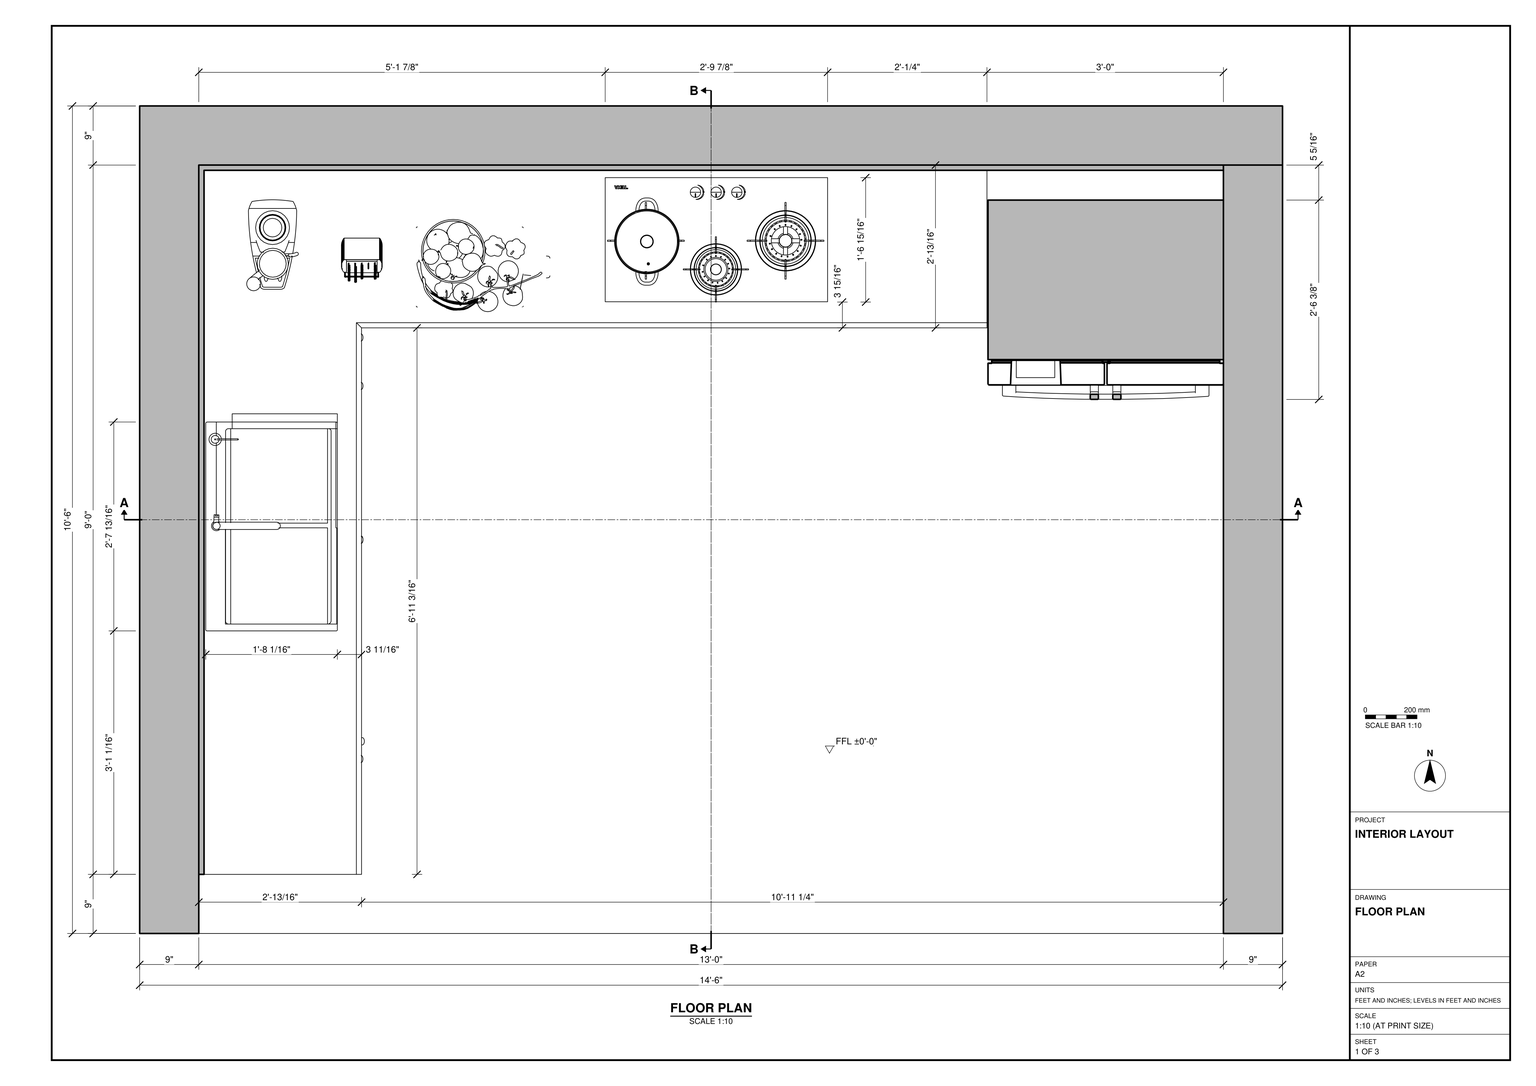
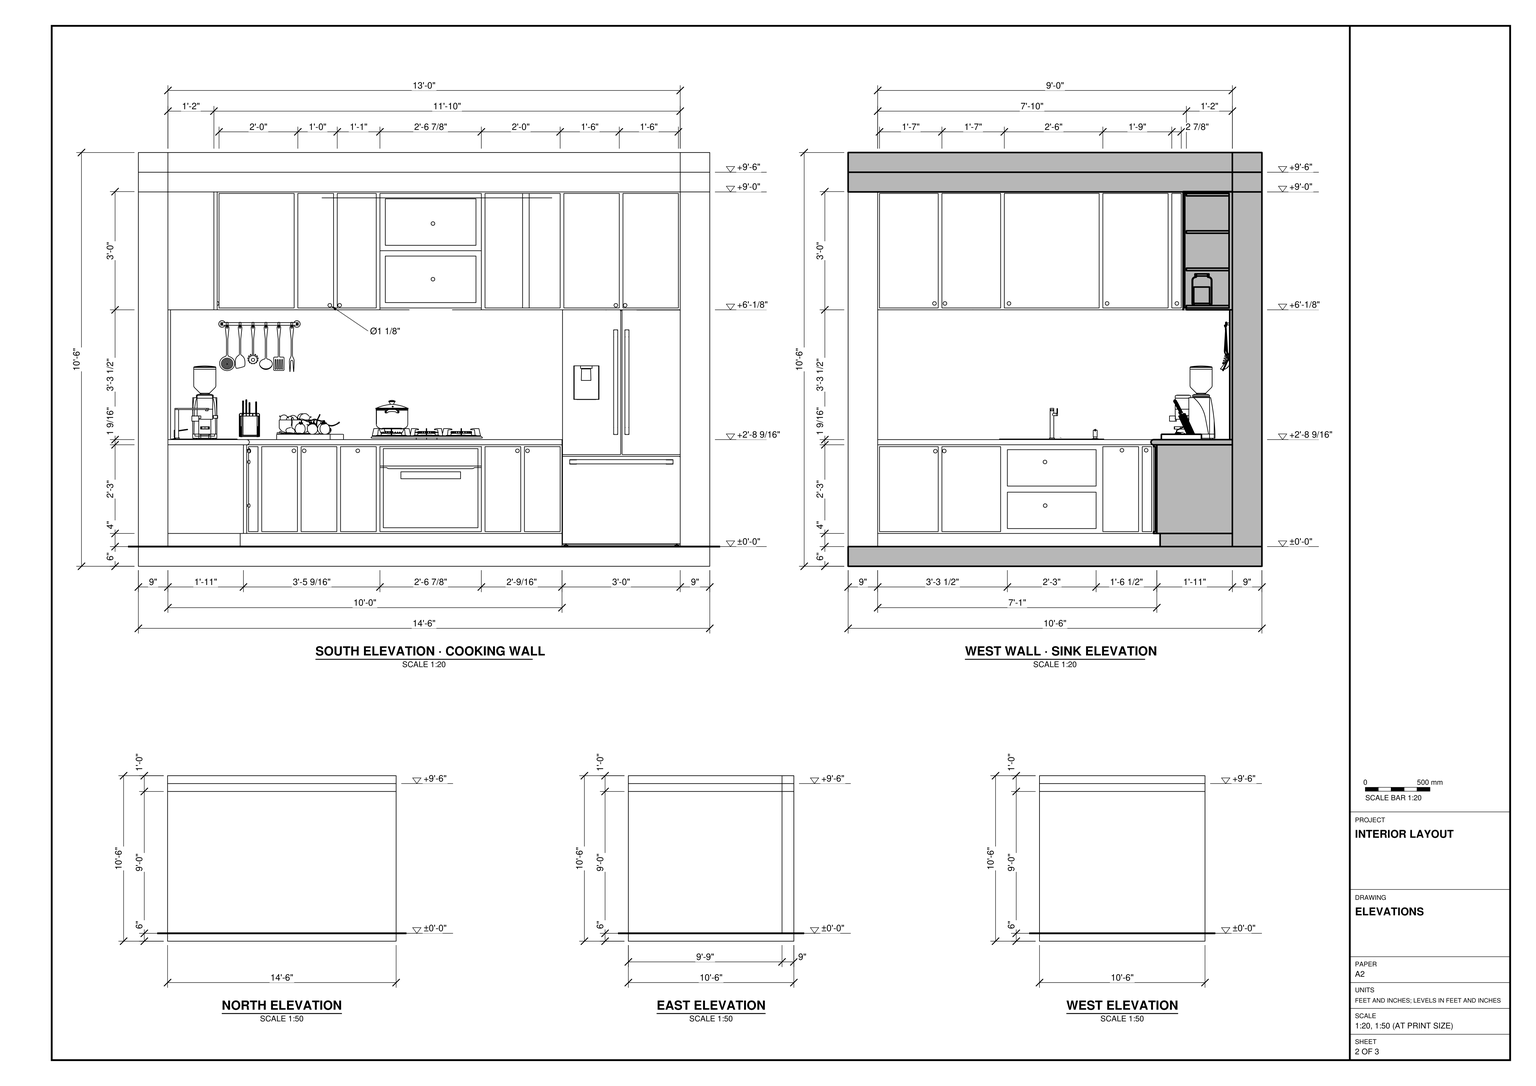
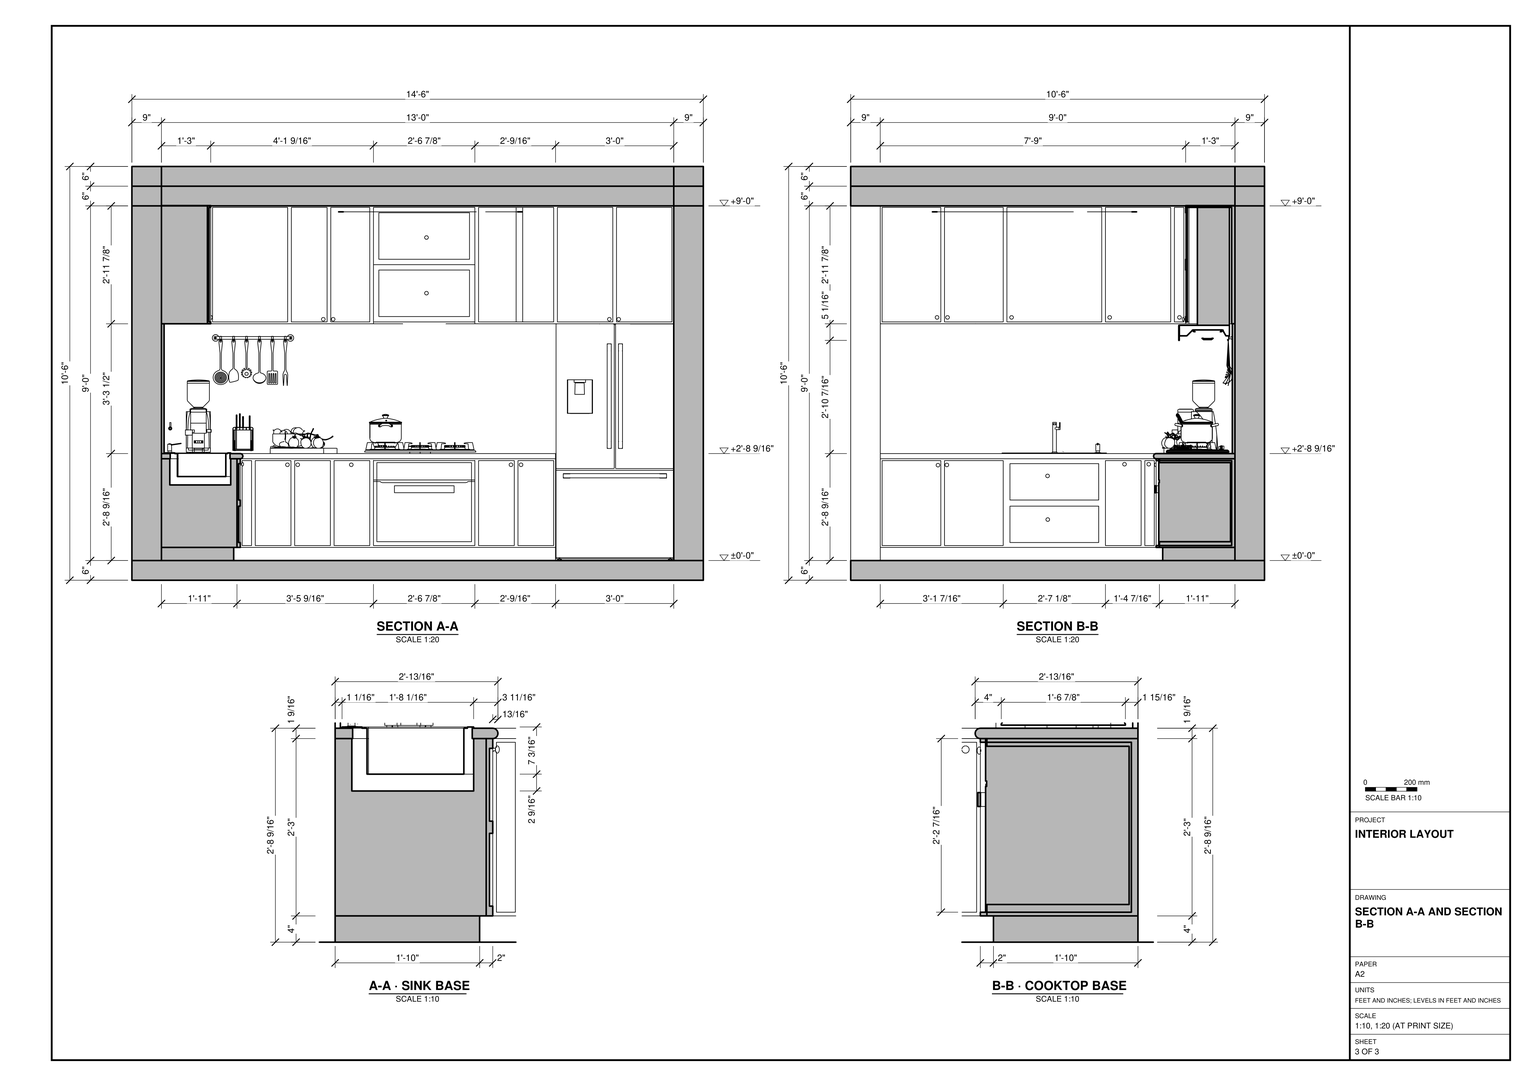
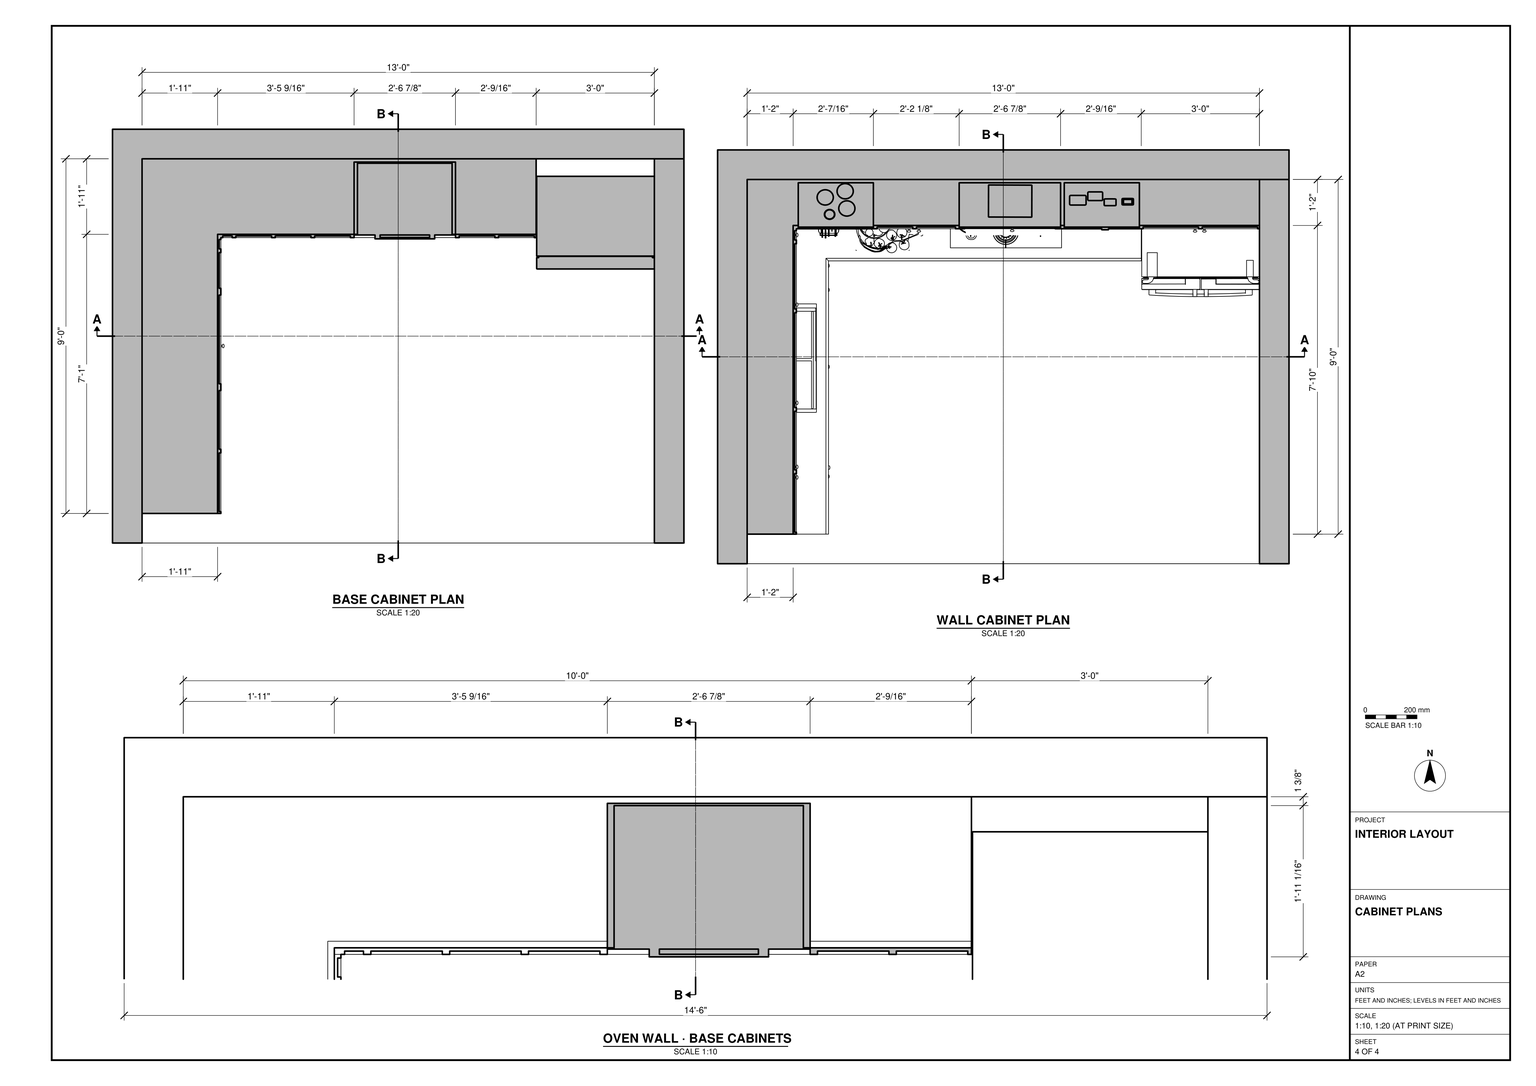
Build the kitchen interior in SketchUp from task_files/diagram_01.pdf. Work in feet and inches. The overall model is 14'-6" wide, 10'-6" deep and 10'-6" high, with the finished floor at ±0'-0". Model the floor slab, the 9" walls and the overhead slab as shown in section. Leave the front open as shown in plan.

Fit an L-shaped worktop along the cooking wall and the left-hand sink wall, leaving the middle of the room clear. Set the double-bowl sink and faucet into the return. On the cooking wall, place the cooktop over the built-in oven and end the run with the refrigerator on the right. Follow the elevations for the widths and arrangement of cabinet doors, drawer fronts and overhead cupboards, including the cupboard above the refrigerator. Use the enlarged sections for the worktop edges, cabinet depths and recessed plinths.

Decor and loose items, including appliances, cookware and counter accessories, may be any suitable library components placed as shown. Keep the shell elements and each furniture or joinery piece in separate groups or components, and use components for repeated parts. Save one SketchUp model as output_files/l_shaped_kitchen_with_fitted_cabinetry_and_appliances.skp.

# SketchUp Ruby script. Lengths in inches.
U = 1.inch
M = Sketchup.active_model
def pt(a) = Geom::Point3d.new(a.map { |v| v * U })
def face(e, loops, mat)
  f = e.add_face(loops[0].map { |a| pt(a) })
  loops[1..].each { |l| e.add_face(l.map { |a| pt(a) }).erase! }
  f.material = f.back_material = mat if mat
  f
end
# faces: each face lists its corners as indices into pts; further lists are holes
def faces(e, pts, list, mat = nil) = list.each { |f| face(e, (f[0].is_a?(Array) ? f : [f]).map { |l| l.map { |i| pts[i] } }, mat) }
# xy, xz, yz: faces in a plane at the given z, y or x. An outline is a flat list of corners, or four numbers for a rectangle; further outlines are holes
def ring(l) = l.size == 4 ? [[l[0], l[1]], [l[2], l[1]], [l[2], l[3]], [l[0], l[3]]] : l.each_slice(2).to_a
def flat(e, list, mat, &to3) = list.each { |f| face(e, (f[0].is_a?(Array) ? f : [f]).map { |l| ring(l).map { |u, v| to3.(u, v) } }, mat) }
def xy(e, z, list, mat = nil) = flat(e, list, mat) { |x, y| [x, y, z] }
def xz(e, y, list, mat = nil) = flat(e, list, mat) { |x, z| [x, y, z] }
def yz(e, x, list, mat = nil) = flat(e, list, mat) { |y, z| [x, y, z] }
def lines(e, pts, list) = list.each { |a, b| e.add_line(pt(pts[a]), pt(pts[b])) }
# prism: a flat outline (further loops are holes) pulled along v
def prism(e, loops, v, mat = nil)
  f = face(e, loops, mat); d = Geom::Vector3d.new(v.map { |x| x * U })
  f.pushpull(f.normal.samedirection?(d) ? d.length : -d.length)
end
def box(e, o, s, mat = nil) = prism(e, [[o, [o[0] + s[0], o[1], o[2]], [o[0] + s[0], o[1] + s[1], o[2]], [o[0], o[1] + s[1], o[2]]]], [0, 0, s[2]], mat)
def at(x, y, z, deg = 0) = Geom::Transformation.translation(pt([x, y, z])) * Geom::Transformation.rotation(ORIGIN, Z_AXIS, deg.degrees)
def axes(o, x, y, z) = Geom::Transformation.new([*x, 0, *y, 0, *z, 0, *pt(o).to_a, 1])
def part(name) = M.definitions.add(name)
# library, detail: a bought-in or finely detailed component or shape, given as its bounding box
def library(name, o, s) = part(name).tap { |d| box(d.entities, o, s) }
def detail(e, o, s) = box(e.add_group.entities, o, s)
def put(e, d, t, mat = nil) = e.add_instance(d, t).tap { |i| i.material = mat if mat }
def group(e, t, mat = nil) = e.add_group.tap { |g| g.transformation = t; g.material = mat if mat }.entities
root = M.entities
M.materials.add("2037 AP 8775 ROCK CRYSTAL").color = [151, 134, 122]
M.materials.add("Crazing Tile_ Stack (YETCY4)").color = [230, 230, 227]
M.materials.add("Granite (R3V8QC)").color = [36, 36, 36]
M.materials.add("Grey Victorian Tile Stack 912 x 912 mm (XTX9T6)").color = [186, 184, 188]
M.materials.add("H 6800 BM").color = [58, 58, 58]
M.materials.add("LED_3200k\#1").color = [255, 192, 121]
M.materials.add("OJ0111").color = [63, 63, 63]
M.materials.add("OJ0113").color = [243, 243, 243]
M.materials.add("OJ0114").color = [42, 42, 42]
M.materials.add("Porphyritic Granite (I3ZB3U)").color = [204, 204, 204]
M.materials.add("[Color A02]").color = [134, 143, 158]
M.materials.add("[Color M01]").color = [226, 226, 226]
M.materials.add("[Translucent Glass Gray]").color = [128, 128, 128]
M.materials["[Translucent Glass Gray]"].alpha = 0.5
c1 = library("H 6800 BM",[0,-1.38,0],[23.62,23.03,17.72])
c2 = part("Component")
xy(c2.entities,-0.07,[[484.96,-0.56,484.96,6.6,485.72,-0.48],[485.72,-0.48,484.96,6.6,486.42,-0.24],[486.42,-0.24,484.96,6.6,487.04,0.14],[487.04,0.14,484.96,6.6,487.55,0.63],[487.55,0.63,484.96,6.6,487.95,1.22],
  [487.95,1.22,484.96,6.6,488.2,1.88],[488.2,1.88,484.96,6.6,488.29,2.61],[488.29,2.61,484.96,6.6,488.29,3.43],[488.29,3.43,484.96,6.6,485.72,6.51],[488.29,3.43,485.72,6.51,488.2,4.15],
  [488.2,4.15,485.72,6.51,487.95,4.82],[487.95,4.82,485.72,6.51,486.42,6.27],[487.95,4.82,486.42,6.27,487.55,5.41],[487.55,5.41,486.42,6.27,487.04,5.9]],"OJ0113")
xy(c2.entities,0.03,[[484.96,-0.56,485.72,-0.48,484.96,6.6],[485.72,-0.48,486.42,-0.24,484.96,6.6],[486.42,-0.24,487.04,0.14,484.96,6.6],[487.04,0.14,487.55,0.63,484.96,6.6],[487.55,0.63,487.95,1.22,484.96,6.6],
  [487.95,1.22,488.2,1.88,484.96,6.6],[488.2,1.88,488.29,2.61,484.96,6.6],[488.29,2.61,488.29,3.43,484.96,6.6],[488.29,3.43,485.72,6.51,484.96,6.6],[488.29,3.43,488.2,4.15,485.72,6.51],
  [488.2,4.15,487.95,4.82,485.72,6.51],[487.95,4.82,486.42,6.27,485.72,6.51],[487.95,4.82,487.55,5.41,486.42,6.27],[487.55,5.41,487.04,5.9,486.42,6.27]],"OJ0113")
xy(c2.entities,0.14,[[-352.59,-0.56,-353.35,-0.48,-355.91,2.61],[-352.59,-0.56,-355.91,2.61,-355.91,3.43],[-353.35,-0.48,-354.05,-0.24,-355.91,2.61],[-354.05,-0.24,-354.67,0.14,-355.91,2.61],[-354.67,0.14,-355.18,0.63,-355.91,2.61],
  [-355.18,0.63,-355.58,1.22,-355.91,2.61],[-355.58,1.22,-355.83,1.88,-355.91,2.61]],"OJ0113")
xy(c2.entities,0.24,[[-352.59,-0.56,-355.91,2.61,-353.35,-0.48],[-352.59,-0.56,-355.91,3.43,-355.91,2.61],[-353.35,-0.48,-355.91,2.61,-354.05,-0.24],[-354.05,-0.24,-355.91,2.61,-354.67,0.14],[-354.67,0.14,-355.91,2.61,-355.18,0.63],
  [-355.18,0.63,-355.91,2.61,-355.58,1.22],[-355.58,1.22,-355.91,2.61,-355.83,1.88]],"OJ0113")
xz(c2.entities,-0.56,[[484.96,-0.07,484.96,0.03,-352.59,0.14],[484.96,0.03,-352.59,0.24,-352.59,0.14]],"OJ0113")
xz(c2.entities,6.6,[[484.96,-0.07,-352.59,0.14,-352.59,0.24],[484.96,-0.07,-352.59,0.24,484.96,0.03]],"OJ0113")
yz(c2.entities,-355.91,[[2.61,0.14,2.61,0.24,3.43,0.14],[3.43,0.14,2.61,0.24,3.43,0.24]],"OJ0113")
yz(c2.entities,488.29,[[2.61,-0.07,3.43,-0.07,3.43,0.03],[2.61,-0.07,3.43,0.03,2.61,0.03]],"OJ0113")
p = [[-355.91,3.43,0.14],[-355.83,4.15,0.14],[484.96,-0.56,-0.07],[-352.59,-0.56,0.14],[-355.58,4.82,0.14],[-355.18,5.41,0.14],
  [-354.67,5.9,0.14],[-354.05,6.27,0.14],[-353.35,6.51,0.14],[-352.59,6.6,0.14],[484.96,6.6,-0.07],[485.72,-0.48,0.03],
  [484.96,-0.56,0.03],[485.72,-0.48,-0.07],[486.42,-0.24,0.03],[486.42,-0.24,-0.07],[487.04,0.14,0.03],[487.04,0.14,-0.07],
  [487.55,0.63,0.03],[487.55,0.63,-0.07],[487.95,1.22,0.03],[487.95,1.22,-0.07],[488.2,1.88,0.03],[488.2,1.88,-0.07],
  [488.29,2.61,0.03],[488.29,2.61,-0.07],[488.2,4.15,0.03],[488.29,3.43,0.03],[488.29,3.43,-0.07],[488.2,4.15,-0.07],
  [487.95,4.82,0.03],[487.95,4.82,-0.07],[487.55,5.41,0.03],[487.55,5.41,-0.07],[487.04,5.9,0.03],[487.04,5.9,-0.07],
  [486.42,6.27,0.03],[486.42,6.27,-0.07],[485.72,6.51,0.03],[485.72,6.51,-0.07],[484.96,6.6,0.03],[-355.83,4.15,0.24],
  [-355.91,3.43,0.24],[-352.59,-0.56,0.24],[-355.58,4.82,0.24],[-355.18,5.41,0.24],[-354.67,5.9,0.24],[-354.05,6.27,0.24],
  [-353.35,6.51,0.24],[-352.59,6.6,0.24],[-353.35,-0.48,0.24],[-353.35,-0.48,0.14],[-354.05,-0.24,0.24],[-354.05,-0.24,0.14],
  [-354.67,0.14,0.24],[-354.67,0.14,0.14],[-355.18,0.63,0.24],[-355.18,0.63,0.14],[-355.58,1.22,0.24],[-355.58,1.22,0.14],
  [-355.83,1.88,0.24],[-355.83,1.88,0.14],[-355.91,2.61,0.24],[-355.91,2.61,0.14]]
faces(c2.entities,p,[[0,1,2],[0,2,3],[1,4,2],[4,5,2],[5,6,2],[6,7,2],[7,8,2],[8,9,2],
  [9,10,2],[11,12,2],[2,13,11],[14,11,13],[13,15,14],[16,14,15],[15,17,16],[18,16,17],
  [17,19,18],[20,18,19],[19,21,20],[22,20,21],[21,23,22],[24,22,23],[23,25,24],[26,27,28],
  [28,29,26],[30,26,29],[29,31,30],[32,30,31],[31,33,32],[34,32,33],[33,35,34],[36,34,35],
  [35,37,36],[38,36,37],[37,39,38],[40,38,39],[39,10,40],[12,41,42],[43,12,42],[12,44,41],
  [12,45,44],[12,46,45],[12,47,46],[12,48,47],[12,49,48],[12,40,49],[43,50,51],[51,3,43],
  [50,52,53],[53,51,50],[52,54,55],[55,53,52],[54,56,57],[57,55,54],[56,58,59],[59,57,56],
  [58,60,61],[61,59,58],[60,62,63],[63,61,60],[42,41,1],[1,0,42],[41,44,4],[4,1,41],
  [44,45,5],[5,4,44],[45,46,6],[6,5,45],[46,47,7],[7,6,46],[47,48,8],[8,7,47],
  [48,49,9],[9,8,48]],"OJ0113")
c3 = library("Component4\#1",[-96.69,-0.16,-6.85],[188.82,0.26,19.29])
c4 = library("Component21",[-484.32,-250.11,-18.2],[1101.05,500.18,71.65])
c5 = part("Component22")
xy(c5.entities,3.45,[[-195,-160.05,-197.98,-159.49,-121.02,-160.03],[-121.02,-160.03,-199.77,-157.83,-200.36,-155.05],[-121.02,-160.03,-200.36,-155.05,-121,-96.03],[-121.02,-160.03,-197.98,-159.49,-199.77,-157.83],[-121.02,-160.03,-121,-96.03,-41.66,-96.01],
  [-121.02,-160.03,-41.66,-96.01,-41.67,-160.01],[174.2,-160.02,-41.67,-160.01,174.21,-96.02],[174.2,-160.02,174.21,-96.02,253.56,-96.01],[174.2,-160.02,253.56,-96.01,253.54,-160.01],[-41.67,-160.01,-41.66,-96.01,174.21,-96.02],
  [253.54,-160.01,253.56,-96.01,332.9,-95.99],[253.54,-160.01,332.9,-95.99,327.53,-159.99],[327.53,-159.99,332.9,-95.99,330.5,-159.44],[330.5,-159.44,332.9,-95.99,332.29,-157.77],[332.29,-157.77,332.9,-95.99,332.89,-154.99],
  [-200.36,-155.05,-200.35,-96.05,-121,-96.03],[-200.35,-96.05,-120.99,-32.03,-121,-96.03],[-200.35,-96.05,-200.34,-32.05,-120.99,-32.03],[-121,-96.03,-120.99,-32.03,-41.64,-32.01],[-121,-96.03,-41.64,-32.01,-41.66,-96.01],
  [174.21,-96.02,-41.66,-96.01,174.23,-32.02],[174.21,-96.02,174.23,-32.02,253.57,-32.01],[174.21,-96.02,253.57,-32.01,253.56,-96.01],[-41.66,-96.01,-41.64,-32.01,174.23,-32.02],[253.56,-96.01,253.57,-32.01,332.92,-31.99],
  [253.56,-96.01,332.92,-31.99,332.9,-95.99],[-200.34,-32.05,-120.98,31.97,-120.99,-32.03],[-200.34,-32.05,-200.32,31.95,-120.98,31.97],[-120.99,-32.03,-120.98,31.97,-41.63,31.99],[-120.99,-32.03,-41.63,31.99,-41.64,-32.01],
  [174.23,-32.02,-41.64,-32.01,174.24,31.98],[174.23,-32.02,174.24,31.98,253.59,31.99],[174.23,-32.02,253.59,31.99,253.57,-32.01],[-41.64,-32.01,-41.63,31.99,174.24,31.98],[253.57,-32.01,253.59,31.99,332.93,32.01],
  [253.57,-32.01,332.93,32.01,332.92,-31.99],[-200.32,31.95,-120.96,95.97,-120.98,31.97],[-200.32,31.95,-200.31,95.95,-120.96,95.97],[-120.98,31.97,-120.96,95.97,-41.62,95.99],[-120.98,31.97,-41.62,95.99,-41.63,31.99],
  [174.24,31.98,-41.63,31.99,174.25,95.98],[174.24,31.98,174.25,95.98,253.6,95.99],[174.24,31.98,253.6,95.99,253.59,31.99],[-41.63,31.99,-41.62,95.99,174.25,95.98],[253.59,31.99,253.6,95.99,332.94,96.01],
  [253.59,31.99,332.94,96.01,332.93,32.01],[-200.31,95.95,-120.95,159.97,-120.96,95.97],[-200.31,95.95,-194.93,159.95,-120.95,159.97],[-200.31,95.95,-197.91,159.4,-194.93,159.95],[-200.31,95.95,-199.7,157.73,-197.91,159.4],
  [-200.31,95.95,-200.29,154.95,-199.7,157.73],[-120.96,95.97,-120.95,159.97,-41.6,159.99],[-120.96,95.97,-41.6,159.99,-41.62,95.99],[174.25,95.98,-41.62,95.99,174.27,159.98],[174.25,95.98,174.27,159.98,253.61,159.99],
  [174.25,95.98,253.61,159.99,253.6,95.99],[-41.62,95.99,-41.6,159.99,174.27,159.98],[253.6,95.99,253.61,159.99,332.96,155.01],[253.6,95.99,332.96,155.01,332.94,96.01],[332.96,155.01,253.61,159.99,332.36,157.79],
  [332.36,157.79,253.61,159.99,330.58,159.45],[330.58,159.45,253.61,159.99,327.6,160.01]],"OJ0111")
xy(c5.entities,805.65,[[-195,-160.05,-121,-96.03,-200.35,-96.05],[-195,-160.05,-200.35,-96.05,-197.98,-159.49],[-195,-160.05,-121.02,-160.03,-121,-96.03],[-121.02,-160.03,-41.66,-96.01,-121,-96.03],[-121.02,-160.03,-41.67,-160.01,-41.66,-96.01],
  [174.2,-160.02,174.21,-96.02,-41.67,-160.01],[174.2,-160.02,253.54,-160.01,253.56,-96.01],[174.2,-160.02,253.56,-96.01,174.21,-96.02],[-41.67,-160.01,174.21,-96.02,-41.66,-96.01],[253.54,-160.01,327.53,-159.99,330.5,-159.44],
  [253.54,-160.01,330.5,-159.44,332.29,-157.77],[253.54,-160.01,332.29,-157.77,332.89,-154.99],[253.54,-160.01,332.89,-154.99,332.9,-95.99],[253.54,-160.01,332.9,-95.99,253.56,-96.01],[-197.98,-159.49,-200.35,-96.05,-199.77,-157.83],
  [-199.77,-157.83,-200.35,-96.05,-200.36,-155.05],[-200.35,-96.05,-120.99,-32.03,-200.34,-32.05],[-200.35,-96.05,-121,-96.03,-120.99,-32.03],[-121,-96.03,-41.64,-32.01,-120.99,-32.03],[-121,-96.03,-41.66,-96.01,-41.64,-32.01],
  [174.21,-96.02,174.23,-32.02,-41.66,-96.01],[174.21,-96.02,253.56,-96.01,253.57,-32.01],[174.21,-96.02,253.57,-32.01,174.23,-32.02],[-41.66,-96.01,174.23,-32.02,-41.64,-32.01],[253.56,-96.01,332.9,-95.99,332.92,-31.99],
  [253.56,-96.01,332.92,-31.99,253.57,-32.01],[-200.34,-32.05,-120.98,31.97,-200.32,31.95],[-200.34,-32.05,-120.99,-32.03,-120.98,31.97],[-120.99,-32.03,-41.63,31.99,-120.98,31.97],[-120.99,-32.03,-41.64,-32.01,-41.63,31.99],
  [174.23,-32.02,174.24,31.98,-41.64,-32.01],[174.23,-32.02,253.57,-32.01,253.59,31.99],[174.23,-32.02,253.59,31.99,174.24,31.98],[-41.64,-32.01,174.24,31.98,-41.63,31.99],[253.57,-32.01,332.92,-31.99,332.93,32.01],
  [253.57,-32.01,332.93,32.01,253.59,31.99],[-200.32,31.95,-120.96,95.97,-200.31,95.95],[-200.32,31.95,-120.98,31.97,-120.96,95.97],[-120.98,31.97,-41.62,95.99,-120.96,95.97],[-120.98,31.97,-41.63,31.99,-41.62,95.99],
  [174.24,31.98,174.25,95.98,-41.63,31.99],[174.24,31.98,253.59,31.99,253.6,95.99],[174.24,31.98,253.6,95.99,174.25,95.98],[-41.63,31.99,174.25,95.98,-41.62,95.99],[253.59,31.99,332.93,32.01,332.94,96.01],
  [253.59,31.99,332.94,96.01,253.6,95.99],[-200.31,95.95,-120.95,159.97,-200.29,154.95],[-200.31,95.95,-120.96,95.97,-120.95,159.97],[-120.96,95.97,-41.6,159.99,-120.95,159.97],[-120.96,95.97,-41.62,95.99,-41.6,159.99],
  [174.25,95.98,174.27,159.98,-41.62,95.99],[174.25,95.98,253.6,95.99,253.61,159.99],[174.25,95.98,253.61,159.99,174.27,159.98],[-41.62,95.99,174.27,159.98,-41.6,159.99],[253.6,95.99,327.6,160.01,253.61,159.99],
  [253.6,95.99,332.94,96.01,327.6,160.01],[332.94,96.01,330.58,159.45,327.6,160.01],[332.94,96.01,332.36,157.79,330.58,159.45],[332.94,96.01,332.96,155.01,332.36,157.79],[-200.29,154.95,-120.95,159.97,-199.7,157.73],
  [-199.7,157.73,-120.95,159.97,-197.91,159.4],[-197.91,159.4,-120.95,159.97,-194.93,159.95]],"OJ0111")
p = [[-195,-160.05,103.64],[-197.98,-159.49,103.64],[-197.98,-159.49,3.45],[-195,-160.05,3.45],[-121.02,-160.03,103.64],[-121.02,-160.03,3.45],
  [-41.67,-160.01,103.64],[-41.67,-160.01,3.45],[174.2,-160.02,103.64],[174.2,-160.02,3.45],[253.54,-160.01,103.64],[253.54,-160.01,3.45],
  [327.53,-159.99,103.64],[327.53,-159.99,3.45],[330.5,-159.44,3.45],[330.5,-159.44,103.64],[-199.77,-157.83,103.64],[-199.77,-157.83,3.45],
  [332.29,-157.77,3.45],[332.29,-157.77,103.64],[-200.36,-155.05,103.64],[-200.36,-155.05,3.45],[332.89,-154.99,3.45],[332.89,-154.99,103.64],
  [-200.35,-96.05,103.64],[-200.35,-96.05,3.45],[332.9,-95.99,103.64],[332.9,-95.99,3.45],[-200.34,-32.05,103.64],[-200.34,-32.05,3.45],
  [332.92,-31.99,103.64],[332.92,-31.99,3.45],[-200.32,31.95,103.64],[-200.32,31.95,3.45],[332.93,32.01,103.64],[332.93,32.01,3.45],
  [-200.31,95.95,103.64],[-200.31,95.95,3.45],[332.94,96.01,103.64],[332.94,96.01,3.45],[-200.29,154.95,103.64],[-200.29,154.95,3.45],
  [332.96,155.01,103.64],[332.96,155.01,3.45],[-199.7,157.73,3.45],[-199.7,157.73,103.64],[332.36,157.79,3.45],[332.36,157.79,103.64],
  [-197.91,159.4,3.45],[-197.91,159.4,103.64],[330.58,159.45,3.45],[330.58,159.45,103.64],[-194.93,159.95,3.45],[-194.93,159.95,103.64],
  [327.6,160.01,3.45],[327.6,160.01,103.64],[-120.95,159.97,103.64],[-120.95,159.97,3.45],[-41.6,159.99,103.64],[-41.6,159.99,3.45],
  [174.27,159.98,103.64],[174.27,159.98,3.45],[253.61,159.99,103.64],[253.61,159.99,3.45],[-195,-160.05,203.82],[-197.98,-159.49,203.82],
  [-121.02,-160.03,203.82],[-41.67,-160.01,203.82],[174.2,-160.02,203.82],[253.54,-160.01,203.82],[327.53,-159.99,203.82],[330.5,-159.44,203.82],
  [-199.77,-157.83,203.82],[332.29,-157.77,203.82],[-200.36,-155.05,203.82],[332.89,-154.99,203.82],[-200.35,-96.05,203.82],[332.9,-95.99,203.82],
  [-200.34,-32.05,203.82],[332.92,-31.99,203.82],[-200.32,31.95,203.82],[332.93,32.01,203.82],[-200.31,95.95,203.82],[332.94,96.01,203.82],
  [-200.29,154.95,203.82],[332.96,155.01,203.82],[-199.7,157.73,203.82],[332.36,157.79,203.82],[-197.91,159.4,203.82],[330.58,159.45,203.82],
  [-194.93,159.95,203.82],[327.6,160.01,203.82],[-120.95,159.97,203.82],[-41.6,159.99,203.82],[174.27,159.98,203.82],[253.61,159.99,203.82],
  [-195,-160.05,304],[-197.98,-159.49,304],[-121.02,-160.03,304],[-41.67,-160.01,304],[174.2,-160.02,304],[253.54,-160.01,304],
  [327.53,-159.99,304],[330.5,-159.44,304],[-199.77,-157.83,304],[332.29,-157.77,304],[-200.36,-155.05,304],[332.89,-154.99,304],
  [-200.35,-96.05,304],[332.9,-95.99,304],[-200.34,-32.05,304],[332.92,-31.99,304],[-200.32,31.95,304],[332.93,32.01,304],
  [-200.31,95.95,304],[332.94,96.01,304],[-200.29,154.95,304],[332.96,155.01,304],[-199.7,157.73,304],[332.36,157.79,304],
  [-197.91,159.4,304],[330.58,159.45,304],[-194.93,159.95,304],[327.6,160.01,304],[-120.95,159.97,304],[-41.6,159.99,304],
  [174.27,159.98,304],[253.61,159.99,304],[-195,-160.05,404.18],[-197.98,-159.49,404.18],[-121.02,-160.03,404.18],[-41.67,-160.01,404.18],
  [174.2,-160.02,404.18],[253.54,-160.01,404.18],[327.53,-159.99,404.18],[330.5,-159.44,404.18],[-199.77,-157.83,404.18],[332.29,-157.77,404.18],
  [-200.36,-155.05,404.18],[332.89,-154.99,404.18],[-200.35,-96.05,404.18],[332.9,-95.99,404.18],[-200.34,-32.05,404.18],[332.92,-31.99,404.18],
  [-200.32,31.95,404.18],[332.93,32.01,404.18],[-200.31,95.95,404.18],[332.94,96.01,404.18],[-200.29,154.95,404.18],[332.96,155.01,404.18],
  [-199.7,157.73,404.18],[332.36,157.79,404.18],[-197.91,159.4,404.18],[330.58,159.45,404.18],[-194.93,159.95,404.18],[327.6,160.01,404.18],
  [-120.95,159.97,404.18],[-41.6,159.99,404.18],[174.27,159.98,404.18],[253.61,159.99,404.18],[-195,-160.05,805.65],[-197.98,-159.49,805.65],
  [-121.02,-160.03,805.65],[-41.67,-160.01,805.65],[174.2,-160.02,805.65],[253.54,-160.01,805.65],[327.53,-159.99,805.65],[330.5,-159.44,805.65],
  [-199.77,-157.83,805.65],[332.29,-157.77,805.65],[-200.36,-155.05,805.65],[332.89,-154.99,805.65],[-200.35,-96.05,805.65],[332.9,-95.99,805.65],
  [-200.34,-32.05,805.65],[332.92,-31.99,805.65],[-200.32,31.95,805.65],[332.93,32.01,805.65],[-200.31,95.95,805.65],[332.94,96.01,805.65],
  [-200.29,154.95,805.65],[332.96,155.01,805.65],[-199.7,157.73,805.65],[332.36,157.79,805.65],[-197.91,159.4,805.65],[330.58,159.45,805.65],
  [-194.93,159.95,805.65],[327.6,160.01,805.65],[-120.95,159.97,805.65],[-41.6,159.99,805.65],[174.27,159.98,805.65],[253.61,159.99,805.65]]
faces(c5.entities,p,[[0,1,2],[2,3,0],[4,0,3],[3,5,4],[6,4,5],[5,7,6],[8,6,7],[7,9,8],
  [10,8,9],[9,11,10],[12,10,11],[11,13,12],[13,14,15],[15,12,13],[1,16,17],[17,2,1],
  [14,18,19],[19,15,14],[16,20,21],[21,17,16],[18,22,23],[23,19,18],[20,24,25],[25,21,20],
  [26,23,22],[22,27,26],[24,28,29],[29,25,24],[30,26,27],[27,31,30],[28,32,33],[33,29,28],
  [34,30,31],[31,35,34],[32,36,37],[37,33,32],[38,34,35],[35,39,38],[36,40,41],[41,37,36],
  [42,38,39],[39,43,42],[44,41,40],[40,45,44],[43,46,47],[47,42,43],[48,44,45],[45,49,48],
  [46,50,51],[51,47,46],[52,48,49],[49,53,52],[50,54,55],[55,51,50],[53,56,57],[57,52,53],
  [56,58,59],[59,57,56],[58,60,61],[61,59,58],[60,62,63],[63,61,60],[62,55,54],[54,63,62],
  [64,65,1],[1,0,64],[66,64,0],[0,4,66],[67,66,4],[4,6,67],[68,67,6],[6,8,68],
  [69,68,8],[8,10,69],[70,69,10],[10,12,70],[12,15,71],[71,70,12],[65,72,16],[16,1,65],
  [15,19,73],[73,71,15],[72,74,20],[20,16,72],[19,23,75],[75,73,19],[74,76,24],[24,20,74],
  [77,75,23],[23,26,77],[76,78,28],[28,24,76],[79,77,26],[26,30,79],[78,80,32],[32,28,78],
  [81,79,30],[30,34,81],[80,82,36],[36,32,80],[83,81,34],[34,38,83],[82,84,40],[40,36,82],
  [85,83,38],[38,42,85],[45,40,84],[84,86,45],[42,47,87],[87,85,42],[49,45,86],[86,88,49],
  [47,51,89],[89,87,47],[53,49,88],[88,90,53],[51,55,91],[91,89,51],[90,92,56],[56,53,90],
  [92,93,58],[58,56,92],[93,94,60],[60,58,93],[94,95,62],[62,60,94],[95,91,55],[55,62,95],
  [96,97,65],[65,64,96],[98,96,64],[64,66,98],[99,98,66],[66,67,99],[100,99,67],[67,68,100],
  [101,100,68],[68,69,101],[102,101,69],[69,70,102],[70,71,103],[103,102,70],[97,104,72],[72,65,97],
  [71,73,105],[105,103,71],[104,106,74],[74,72,104],[73,75,107],[107,105,73],[106,108,76],[76,74,106],
  [109,107,75],[75,77,109],[108,110,78],[78,76,108],[111,109,77],[77,79,111],[110,112,80],[80,78,110],
  [113,111,79],[79,81,113],[112,114,82],[82,80,112],[115,113,81],[81,83,115],[114,116,84],[84,82,114],
  [117,115,83],[83,85,117],[86,84,116],[116,118,86],[85,87,119],[119,117,85],[88,86,118],[118,120,88],
  [87,89,121],[121,119,87],[90,88,120],[120,122,90],[89,91,123],[123,121,89],[122,124,92],[92,90,122],
  [124,125,93],[93,92,124],[125,126,94],[94,93,125],[126,127,95],[95,94,126],[127,123,91],[91,95,127],
  [128,129,97],[97,96,128],[130,128,96],[96,98,130],[131,130,98],[98,99,131],[132,131,99],[99,100,132],
  [133,132,100],[100,101,133],[134,133,101],[101,102,134],[102,103,135],[135,134,102],[129,136,104],[104,97,129],
  [103,105,137],[137,135,103],[136,138,106],[106,104,136],[105,107,139],[139,137,105],[138,140,108],[108,106,138],
  [141,139,107],[107,109,141],[140,142,110],[110,108,140],[143,141,109],[109,111,143],[142,144,112],[112,110,142],
  [145,143,111],[111,113,145],[144,146,114],[114,112,144],[147,145,113],[113,115,147],[146,148,116],[116,114,146],
  [149,147,115],[115,117,149],[118,116,148],[148,150,118],[117,119,151],[151,149,117],[120,118,150],[150,152,120],
  [119,121,153],[153,151,119],[122,120,152],[152,154,122],[121,123,155],[155,153,121],[154,156,124],[124,122,154],
  [156,157,125],[125,124,156],[157,158,126],[126,125,157],[158,159,127],[127,126,158],[159,155,123],[123,127,159],
  [160,161,129],[129,128,160],[162,160,128],[128,130,162],[163,162,130],[130,131,163],[164,163,131],[131,132,164],
  [165,164,132],[132,133,165],[166,165,133],[133,134,166],[134,135,167],[167,166,134],[161,168,136],[136,129,161],
  [135,137,169],[169,167,135],[168,170,138],[138,136,168],[137,139,171],[171,169,137],[170,172,140],[140,138,170],
  [173,171,139],[139,141,173],[172,174,142],[142,140,172],[175,173,141],[141,143,175],[174,176,144],[144,142,174],
  [177,175,143],[143,145,177],[176,178,146],[146,144,176],[179,177,145],[145,147,179],[178,180,148],[148,146,178],
  [181,179,147],[147,149,181],[150,148,180],[180,182,150],[149,151,183],[183,181,149],[152,150,182],[182,184,152],
  [151,153,185],[185,183,151],[154,152,184],[184,186,154],[153,155,187],[187,185,153],[186,188,156],[156,154,186],
  [188,189,157],[157,156,188],[189,190,158],[158,157,189],[190,191,159],[159,158,190],[191,187,155],[155,159,191]],"OJ0111")
c6 = part("Component23")
xz(c6.entities,-33.11,[[616.86,-0.07,616.86,0.93,-484.68,0.11],[-484.68,0.11,616.86,0.93,-484.68,1.11]],"OJ0114")
xz(c6.entities,38.44,[[616.86,-0.07,-484.68,0.11,-484.68,1.11],[616.86,-0.07,-484.68,1.11,616.86,0.93]],"OJ0114")
yz(c6.entities,-484.68,[[-33.11,0.11,-33.11,1.11,38.44,0.11],[38.44,0.11,-33.11,1.11,38.44,1.11]],"OJ0114")
yz(c6.entities,616.86,[[-33.11,-0.07,38.44,-0.07,38.44,0.93],[-33.11,-0.07,38.44,0.93,-33.11,0.93]],"OJ0114")
p = [[616.86,38.44,-0.07],[616.86,-33.11,-0.07],[-484.68,-33.11,0.11],[-484.68,38.44,0.11],[616.86,38.44,0.93],[-484.68,38.44,1.11],
  [-484.68,-33.11,1.11],[616.86,-33.11,0.93]]
faces(c6.entities,p,[[0,1,2],[2,3,0],[4,5,6],[6,7,4]],"OJ0114")
c7 = part("Component24")
xz(c7.entities,0.54,[[616.86,-0.07,616.86,0.03,-484.68,0.11],[616.86,0.03,-484.68,0.21,-484.68,0.11]],"OJ0114")
xz(c7.entities,2.59,[[616.86,-0.07,-484.68,0.11,-484.68,0.21],[616.86,-0.07,-484.68,0.21,616.86,0.03]],"OJ0114")
yz(c7.entities,-484.68,[[0.54,0.11,0.54,0.21,2.59,0.11],[2.59,0.11,0.54,0.21,2.59,0.21]],"OJ0114")
yz(c7.entities,616.86,[[0.54,-0.07,2.59,-0.07,2.59,0.03],[0.54,-0.07,2.59,0.03,0.54,0.03]],"OJ0114")
p = [[616.86,2.59,-0.07],[616.86,0.54,-0.07],[-484.68,0.54,0.11],[-484.68,2.59,0.11],[616.86,2.59,0.03],[-484.68,2.59,0.21],
  [-484.68,0.54,0.21],[616.86,0.54,0.03]]
faces(c7.entities,p,[[0,1,2],[2,3,0],[4,5,6],[6,7,4]],"OJ0114")
c8 = library("Component25",[-484.68,-48.78,-0.07],[1101.54,102.23,5.18])
c9 = library("Component26",[-251.62,-133.84,-6.74],[635.66,306.9,64.49])
c10 = part("Component2\#1")
put(c10.entities,c2,axes([2.48,-260.87,-470.03],[1.03982,-0.00322,0],[0,0,0.66878],[-0.00189,-0.60059,0]))
put(c10.entities,c3,axes([87.5,-261.2,-443.64],[1.03982,-0.00323,0],[0.00079,0.25397,0],[0,0,0.93112]))
put(c10.entities,c4,axes([2.77,3.04,-462.82],[1.03982,-0.00322,0],[0.00325,1.03133,0],[0,0,0.93112]))
put(c10.entities,c5,axes([4.08,95.86,-416.26],[1.03982,-0.00322,0],[0.00325,1.03133,0],[0,0,0.93112]))
put(c10.entities,c6,axes([1.09,-254.79,-449.26],[1.03982,-0.00322,0],[0,0,0.93112],[-0.00325,-1.03133,0]))
put(c10.entities,c7,axes([1.09,-255.65,-495.28],[1.03982,-0.00322,0],[0,0,0.93112],[-0.00325,-1.03133,0]))
put(c10.entities,c8,axes([1.09,-255.71,-463.13],[1.03982,-0.00322,0],[0,0,0.93112],[-0.00325,-1.03133,0]))
put(c10.entities,c9,axes([2.82,16.54,-496.89],[1.03982,-0.00322,0],[0.00325,1.03133,0],[0,0,0.93112]))
c11 = library("white+sink",[101.38,33.55,27.24],[20.87,33.46,17.21])
c12 = library("B36CD50SNS_tradeCAD",[0,0,0],[35.84,30.35,69.65])
c13 = library("Encurtidos",[-8.17,-2.25,0],[16.27,5.07,6.57])
c14 = library("Spices",[56.83,45.46,21.83],[22.8,4.6,10.33])
c15 = library("Spice Bottles 1b",[-1,-1,0],[14.78,2,4.4])
c16 = library("sj+spices",[21.17,26.0625,-0.02],[21.35,8.125,10.24])
c17 = library("flour+and+oats",[12.67,6.32,0.1],[12.91,12.87,9.32])
c18 = library("Spices\#1",[-1.58,-1.74,0],[7.65,3.48,9.84])
c19 = library("Grinder",[0.01,0,0],[7.86,13.86,22.44])
c20 = library("skpD5F4",[0,-2.85,-0.14],[24.79,2.85,15.53])
c21 = library("Cutlery",[4.03,-1.8,0.87],[6.79,6.23,11.32])
c22 = library("Tabua com vegetais",[0,0,0],[14.04,20.35,7.9375])
c23 = library("Cabinet Knob",[-0.78,-1.58,0],[1.56,1.58,1.5625])
c24 = part("Component\#340")
xy(c24.entities,0,[[35,0,17.5,17.5,18.21,18.21,18.91,17.51,35,1.41,46.14,12.56,46.84,13.26,51.79,8.31,51.09,7.61,50.28,8.43,46.85,11.85],[9.73,16.79,9.01,17.5,13.26,21.74,0,35,11.85,46.85,12.56,46.14,1.41,35,9.03,27.39,9.73,26.6875,13.26,23.16,14.68,21.74],[51.8,16.8,51.09,17.51,51.79,18.21,68.59,35,57.44,46.14,51.79,51.79,56.74,56.74,57.44,56.04,53.2,51.8,70,35],[17.51,51.09,12.56,56.04,13.26,56.74,17.5,52.5,35,70,48.97,56.03,48.26,55.32,35,68.59,18.21,51.79]],"LED_3200k\#1")
c25 = library("Group\#5",[0,9,0],[120,108,28.76])
c26 = library("Group\#6",[0,9,0],[120,108,1.57])
c27 = library("Group\#7",[0,9,0],[97,85,27])
c28 = library("Group\#10",[0,9,0],[142,94,36])
c29 = part("Group\#12")
box(c29.entities,[0,0,0],[22.875,13,0.75])
c30 = part("Group\#14")
box(c30.entities,[0,0,0],[22.875,13,0.75])
c31 = library("Group\#219",[0,0,0],[33.86,18.94,11.96])
c32 = part("Group\#16")
box(c32.entities,[0,-18,0],[174,126,6])
put(root,c1,axes([73.5625,94,10.5625],[1.3071,0,0],[0,1,0],[0,0,1.49229]))
put(root,c10,axes([87.35,107.61,97.49],[0.0238,0,0],[0,0.02956,0],[0,0,0.04807]))
put(root,c11,axes([-87.27,14.1875,5.43],[0.96,0,0],[0,0.9504,0],[0,0,0.96]))
put(root,c12,axes([129.16,81.3125,6],[1,0,0],[0,1,0],[0,0,1.03519]))
put(root,c13,axes([117.34,108.85,79.99],[1.2208,0,0],[0,1.09,0],[0,0,1.09]))
put(root,c14,axes([55.45,66.72,70.49],[0.90922,0,0],[0,0.93,0],[0,0,0.93]))
put(root,c15,axes([108.36,107.18,102.17],[1.4574,0,0],[0,1.1342,0],[0,0,1.44043]))
put(root,c16,axes([1.88,79.9375,79.4375],[1.07132,0,0],[0,0.94,0],[0,0,0.94]))
put(root,c17,axes([18.66,99.39,90.7],[0.91012,0,0],[0,0.8586,0],[0,0,0.8586]))
put(root,c18,at(34.67,110.38,102.17))
put(root,c19,at(24.17,111.72,38.57,-180))
put(root,c20,at(24.48,116.2,59.41))
put(root,c21,at(35.14,95.0625,38.57,90))
put(root,c22,at(42.11,108.72,38.57,-90))
put(root,c23,axes([33.22,29.27,34.5625],[0,0.70998,0],[-0.62416,0,0],[0,0,0.70998]),"[Color M01]")
put(root,c23,axes([33,26.57,34.5],[0,0.70998,0],[-0.62416,0,0],[0,0,0.70998]),"[Color M01]")
put(root,c23,axes([33.01,59.93,31.22],[0,0.70998,0],[-0.62416,0,0],[0,0,0.70998]),"[Color M01]")
put(root,c23,axes([33.01,60,17.93],[0,0.70998,0],[-0.62416,0,0],[0,0,0.70998]),"[Color M01]")
put(root,c23,axes([33.01,83.37,34.78],[0,0.70998,0],[-0.62416,0,0],[0,0,0.70998]),"[Color M01]")
put(root,c23,axes([47.36,93.5,34.61],[0.70998,0,0],[0,0.62416,0],[0,0,0.70998]),"[Color M01]")
put(root,c23,axes([50.49,93.5,34.61],[0.70998,0,0],[0,0.62416,0],[0,0,0.70998]),"[Color M01]")
put(root,c23,axes([66.8,93.5,34.61],[0.70998,0,0],[0,0.62416,0],[0,0,0.70998]),"[Color M01]")
put(root,c23,axes([115.43,93.5,34.61],[0.70998,0,0],[0,0.62416,0],[0,0,0.70998]),"[Color M01]")
put(root,c23,axes([118.49,93.5,34.61],[0.70998,0,0],[0,0.62416,0],[0,0,0.70998]),"[Color M01]")
put(root,c23,axes([23.5,26.29,79.49],[0,0.70998,0],[-0.62416,0,0],[0,0,0.70998]),"[Color M01]")
put(root,c23,axes([23.5,29.48,79.49],[0,0.70998,0],[-0.62416,0,0],[0,0,0.70998]),"[Color M01]")
put(root,c23,axes([23.5,48.98,79.49],[0,0.70998,0],[-0.62416,0,0],[0,0,0.70998]),"[Color M01]")
put(root,c23,axes([23.5,78.85,79.49],[0,0.70998,0],[-0.62416,0,0],[0,0,0.70998]),"[Color M01]")
put(root,c23,axes([23.5,100.1,79.49],[0,0.70998,0],[-0.62416,0,0],[0,0,0.70998]),"[Color M01]")
put(root,c23,axes([33.01,90.75,34.78],[0,0.70998,0],[-0.62416,0,0],[0,0,0.70998]),"[Color M01]")
put(root,c23,axes([58.29,101.9375,78.92],[0.70998,0,0],[0,0.62416,0],[0,0,0.70998]),"[Color M01]")
put(root,c23,axes([61.29,101.9375,78.92],[0.70998,0,0],[0,0.62416,0],[0,0,0.70998]),"[Color M01]")
put(root,c23,axes([89.7,102.1,86.87],[0.70998,0,0],[0,0.62416,0],[0,0,0.70998]),"[Color M01]")
put(root,c23,axes([89.7,102.1,103.8125],[0.70998,0,0],[0,0.62416,0],[0,0,0.70998]),"[Color M01]")
put(root,c23,axes([145.39,101.9375,78.92],[0.70998,0,0],[0,0.62416,0],[0,0,0.70998]),"[Color M01]")
put(root,c23,axes([148.23,101.9375,78.92],[0.70998,0,0],[0,0.62416,0],[0,0,0.70998]),"[Color M01]")
put(root,c24,at(55.91,20.96,112.1875))
g1 = group(root,at(0,18,0))
xy(g1,0,[[0,-18,174,108]])
xy(g1,6,[[0,-18,174,108]],"Grey Victorian Tile Stack 912 x 912 mm (XTX9T6)")
xz(g1,-18,[[0,0,174,6]],"2037 AP 8775 ROCK CRYSTAL")
xz(g1,108,[[0,0,174,6]],"2037 AP 8775 ROCK CRYSTAL")
yz(g1,0,[[-18,0,108,6]],"2037 AP 8775 ROCK CRYSTAL")
yz(g1,174,[[-18,0,108,6]],"2037 AP 8775 ROCK CRYSTAL")
g2 = group(root,at(0,18,6),"2037 AP 8775 ROCK CRYSTAL")
prism(g2,[[[9,99,0],[9,-18,0],[0,-18,0],[0,108,0],[174,108,0],[174,99,0]]],[0,0,120])
g3 = group(root,at(165,18,6),"2037 AP 8775 ROCK CRYSTAL")
box(g3,[0,-18,0],[9,117,120])
g4 = group(root,at(9,0,6),"Granite (R3V8QC)")
prism(g4,[[[22,95,0],[22,9,0],[0,9,0],[0,117,0],[120,117,0],[120,95,0]]],[0,0,4])
put(root,c25,at(9,0,10),"[Color A02]")
put(root,c26,at(9,0,37),"Porphyritic Granite (I3ZB3U)")
put(root,c27,at(32,0,10),"[Color A02]")
g5 = group(root,at(9,0,38.57),"Crazing Tile_ Stack (YETCY4)")
xy(g5,0,[[0,9,0.8,117],[0.8,116.2,156,117]])
xy(g5,39.53,[[0,9,0.8,117],[0.8,116.2,156,117]])
xz(g5,9,[[0,0,0.8,39.53]])
xz(g5,116.2,[[0.8,0,156,39.53]])
xz(g5,117,[[0,24,0.8,39.53],[0.8,24,156,39.53]])
yz(g5,0,[[9,0,117,39.53]])
yz(g5,0.8,[[9,0,116.2,39.53]])
yz(g5,156,[[116.2,0,117,39.53]])
g6 = group(root,at(9,0,78.1),"[Color A02]")
xy(g6,0,[[0,9,14,102],[0,102,0,117,156,117,156,103,95.4375,103,95.4375,116,64.5625,116,64.5625,103,14,103,14,102]])
xy(g6,0.5625,[[15.5625,103,38.4375,116],[96.5625,103,119.4375,116]])
xy(g6,35.4375,[[15.5625,103,38.4375,116],[64.5625,103,95.4375,116],[96.5625,103,119.4375,116]])
xy(g6,36,[[0,9,14,9,14,103,156,103,156,117,0,117]])
xz(g6,9,[[0,0,14,36]])
xz(g6,103,[[[14,0,64.5625,0,64.5625,35.4375,95.4375,35.4375,95.4375,0,156,0,156,36,14,36],[15.5625,0.5625,38.4375,35.4375],[96.5625,0.5625,119.4375,35.4375]]])
xz(g6,116,[[64.5625,0,95.4375,35.4375],[15.5625,0.5625,38.4375,35.4375],[96.5625,0.5625,119.4375,35.4375]])
xz(g6,117,[[0,0,156,36]])
yz(g6,14,[[9,0,103,36]])
yz(g6,15.5625,[[103,0.5625,116,35.4375]])
yz(g6,38.4375,[[103,0.5625,116,35.4375]])
yz(g6,64.5625,[[103,0,116,35.4375]])
yz(g6,95.4375,[[103,0,116,35.4375]])
yz(g6,96.5625,[[103,0.5625,116,35.4375]])
yz(g6,119.4375,[[103,0.5625,116,35.4375]])
yz(g6,156,[[103,0,117,36]])
put(root,c28,at(23,0,78.1),"[Color A02]")
put(root,c29,at(105.5625,103,78.66))
put(root,c29,at(105.5625,103,90.04))
put(root,c29,at(105.5625,103,101.42))
put(root,c29,at(105.5625,103,112.79))
g7 = group(root,at(105.5625,102,78.66),"[Translucent Glass Gray]")
xy(g7,0,[[11.4375,-0.3125,11.4375,0,0,0,0,0.5,22.875,0.5,22.875,0,13.4375,0,13.4375,-0.3125]])
xy(g7,34.875,[[11.4375,-0.3125,13.4375,-0.3125,13.4375,0,22.875,0,22.875,0.5,0,0.5,0,0,11.4375,0]])
xz(g7,-0.3125,[[11.4375,0,13.4375,34.875]],"[Color A02]")
xz(g7,0,[[0,0,11.4375,34.875],[13.4375,0,22.875,34.875]],"[Translucent Glass Gray]")
xz(g7,0.5,[[0,0,22.875,34.875]])
yz(g7,0,[[0,0,0.5,34.875]])
yz(g7,11.4375,[[-0.3125,0,0,34.875]])
yz(g7,13.4375,[[-0.3125,0,0,34.875]])
yz(g7,22.875,[[0,0,0.5,34.875]])
put(root,c30,at(24.5625,103,78.66))
put(root,c30,at(24.5625,103,90.04))
put(root,c30,at(24.5625,103,101.42))
put(root,c30,at(24.5625,103,112.79))
g8 = group(root,at(24.5625,102,78.66),"[Translucent Glass Gray]")
box(g8,[0,0,0],[22.875,0.5,34.875])
put(root,c31,at(104.74,115.09,38.57,180))
g9 = group(root,at(73.5625,102,78.66),"[Color A02]")
xy(g9,0,[[0,0,30.875,0.5]])
xy(g9,1.64,[[1.64,0,29.24,0.3]])
xy(g9,15.8,[[1.64,0,29.24,0.3]])
xy(g9,19.07,[[1.64,0,29.24,0.3]])
xy(g9,33.24,[[1.64,0,29.24,0.3]])
xy(g9,34.875,[[0,0,30.875,0.5]])
xz(g9,0,[[[0,0,30.875,17.4375],[1.64,1.64,29.24,15.8]],[[0,17.4375,30.875,34.875],[1.64,19.07,29.24,33.24]]])
xz(g9,0.3,[[1.64,1.64,29.24,15.8],[1.64,19.07,29.24,33.24]])
xz(g9,0.5,[[0,0,30.875,34.875]])
yz(g9,0,[[0,0,0.5,34.875]])
yz(g9,1.64,[[0,1.64,0.3,15.8],[0,19.07,0.3,33.24]])
yz(g9,29.24,[[0,1.64,0.3,15.8],[0,19.07,0.3,33.24]])
yz(g9,30.875,[[0,0,0.5,34.875]])
g10 = group(root,at(0,0,114),"2037 AP 8775 ROCK CRYSTAL")
put(g10,c32,at(0,18,0),"2037 AP 8775 ROCK CRYSTAL")
put(g10,c32,at(0,18,6),"2037 AP 8775 ROCK CRYSTAL")
